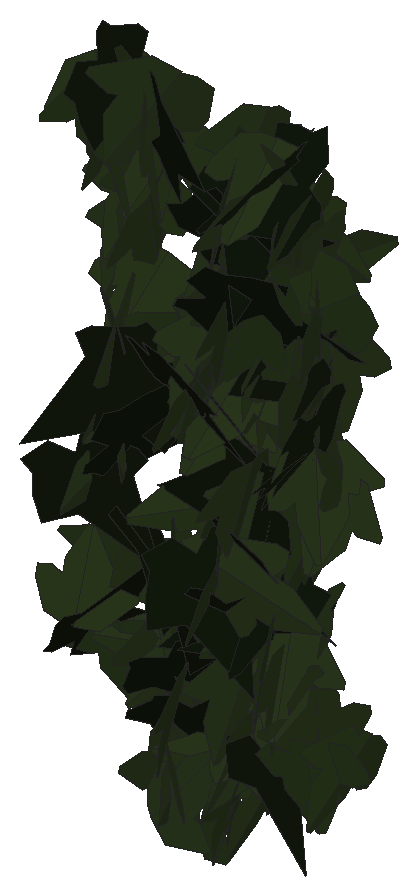
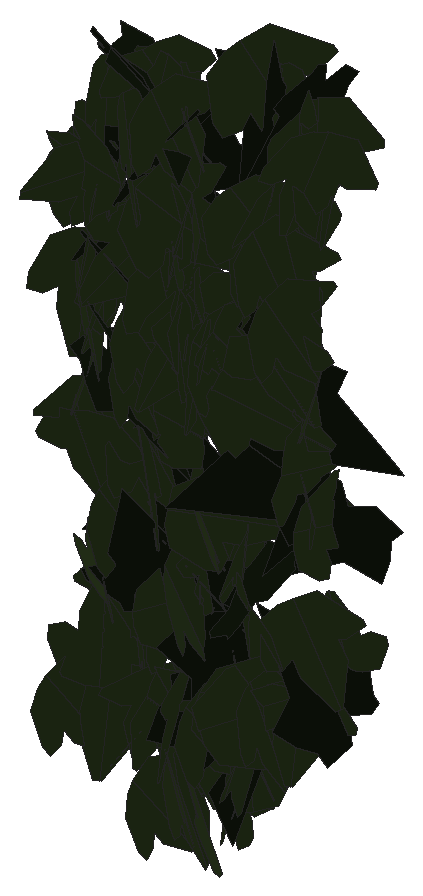
# SketchUp Ruby script. Lengths in inches.
U = 1.inch
M = Sketchup.active_model
def pt(a) = Geom::Point3d.new(a.map { |v| v * U })
def face(e, loops, mat)
  f = e.add_face(loops[0].map { |a| pt(a) })
  loops[1..].each { |l| e.add_face(l.map { |a| pt(a) }).erase! }
  f.material = f.back_material = mat if mat
  f
end
# faces: each face lists its corners as indices into pts; further lists are holes
def faces(e, pts, list, mat = nil) = list.each { |f| face(e, (f[0].is_a?(Array) ? f : [f]).map { |l| l.map { |i| pts[i] } }, mat) }
# xy, xz, yz: faces in a plane at the given z, y or x. An outline is a flat list of corners, or four numbers for a rectangle; further outlines are holes
def ring(l) = l.size == 4 ? [[l[0], l[1]], [l[2], l[1]], [l[2], l[3]], [l[0], l[3]]] : l.each_slice(2).to_a
def flat(e, list, mat, &to3) = list.each { |f| face(e, (f[0].is_a?(Array) ? f : [f]).map { |l| ring(l).map { |u, v| to3.(u, v) } }, mat) }
def xy(e, z, list, mat = nil) = flat(e, list, mat) { |x, y| [x, y, z] }
def xz(e, y, list, mat = nil) = flat(e, list, mat) { |x, z| [x, y, z] }
def yz(e, x, list, mat = nil) = flat(e, list, mat) { |y, z| [x, y, z] }
def lines(e, pts, list) = list.each { |a, b| e.add_line(pt(pts[a]), pt(pts[b])) }
# prism: a flat outline (further loops are holes) pulled along v
def prism(e, loops, v, mat = nil)
  f = face(e, loops, mat); d = Geom::Vector3d.new(v.map { |x| x * U })
  f.pushpull(f.normal.samedirection?(d) ? d.length : -d.length)
end
def box(e, o, s, mat = nil) = prism(e, [[o, [o[0] + s[0], o[1], o[2]], [o[0] + s[0], o[1] + s[1], o[2]], [o[0], o[1] + s[1], o[2]]]], [0, 0, s[2]], mat)
def at(x, y, z, deg = 0) = Geom::Transformation.translation(pt([x, y, z])) * Geom::Transformation.rotation(ORIGIN, Z_AXIS, deg.degrees)
def axes(o, x, y, z) = Geom::Transformation.new([*x, 0, *y, 0, *z, 0, *pt(o).to_a, 1])
def part(name) = M.definitions.add(name)
# library, detail: a bought-in or finely detailed component or shape, given as its bounding box
def library(name, o, s) = part(name).tap { |d| box(d.entities, o, s) }
def detail(e, o, s) = box(e.add_group.entities, o, s)
def put(e, d, t, mat = nil) = e.add_instance(d, t).tap { |i| i.material = mat if mat }
def group(e, t, mat = nil) = e.add_group.tap { |g| g.transformation = t; g.material = mat if mat }.entities
root = M.entities
M.materials.add("efeu1").color = [18, 25, 13]
M.materials.add("efeu2").color = [43, 57, 29]
c1 = part("ivyleaf_9")
p = [[1.54,2.16,1.25],[1.36,2.04,1.19],[-0.21,0.99,0.68],[-0.71,1.11,0.82],[-0.85,0.86,0.67],[-0.8,0.17,0.21],
  [-0.9,-0.01,0.1],[-0.67,-0.16,-0.02],[-0.08,-0.08,-0.05],[-0.03,-0.6,-0.4],[0.65,-0.88,-0.66],[0.83,-0.6,-0.49],
  [1.29,-0.42,-0.43],[1.8125,-0.07,-0.26],[1.21,0.44,0.15]]
faces(c1.entities,p,[[0,1,2,3,4,5,6,7,8,9,10,11,12,13,14]],"efeu1")
c2 = part("ivyleaf_10")
p = [[0,0.5,-0.03],[-0.0625,2.02,-0.43],[-0.19,2.01,-0.46],[-0.54,1.05,-0.29],[-0.52,0.625,-0.18],[-0.83,0.76,-0.28],
  [-1.16,0.64,-0.33],[-1.15,0.33,-0.24],[-0.77,-0.39,0.02],[-0.3,-0.51,0.16],[0.04,-0.48,0.23],[-0.02,2.01,-0.4375],
  [-0.06,2.01,-0.43],[0.04,-0.49,0.23],[0.67,-0.49,0.14],[1.38,0.36,-0.2],[1.375,0.51,-0.24],[0.81,0.65,-0.19],
  [0.62,0.59,-0.15],[0.6,1.09,-0.28],[0.5,1.23,-0.31]]
faces(c2.entities,p,[[0,1,2,3,4,5,6,7,8,9,10],[11,12,0,13,14,15,16,17,18,19,20]],"efeu2")
put(root,c1,axes([509.74,135.35,181.09],[0.74865,0.1371,0.35798],[0.34878,0.0823,-0.76093],[-0.15906,0.82575,0.0164]))
put(root,c2,axes([508.4,135.95,183.89],[-0.44907,-0.51344,0.43661],[-0.29886,-0.31855,-0.682],[0.6041,-0.53928,-0.01283]))
put(root,c2,axes([509.9375,135.84,177.97],[0.03708,-0.698,0.02112],[0.00383,-0.02095,-0.69898],[0.69831,0.03718,0.00271]))
put(root,c1,axes([509.16,135.75,176.39],[0.07993,-0.60102,-0.3989],[-0.03272,0.38262,-0.62961],[0.76932,0.07872,0.01466]))
put(root,c2,axes([509.58,136.01,182.89],[0.42901,-0.54847,0.24214],[0.15092,-0.18937,-0.69632],[0.58024,0.45477,0.00208]))
put(root,c1,axes([508.54,135.55,179.53],[0.80566,-0.10434,-0.13006],[-0.12795,0.02467,-0.81235],[0.10692,0.81571,0.00793]))
put(root,c2,axes([510.26,135.9375,175.45],[0.47005,-0.54569,0.14033],[0.14228,-0.06688,-0.72322],[0.59019,0.45073,0.06259]))
put(root,c1,axes([508.01,136.09,183.3],[0.34957,-0.1483,-0.68391],[0.69592,-0.00675,0.35718],[-0.07361,-0.76804,0.12891]))
put(root,c2,axes([510.26,135.95,183.33],[0.50117,0.37752,-0.27471],[-0.21702,-0.17155,-0.62212],[-0.4478,0.50565,-0.00596]))
put(root,c2,axes([509.875,135.82,176.33],[-0.25449,-0.01854,-0.67596],[0.66869,-0.11431,-0.24861],[-0.10057,-0.71317,0.05742]))
put(root,c2,axes([508.48,135.88,172.03],[0.5067,-0.23136,-0.42913],[0.39952,-0.15767,0.55673],[-0.27941,-0.64501,0.01783]))
put(root,c2,axes([509.73,136.06,174.59],[-0.1443,-0.64865,0.23347],[0.05381,-0.23727,-0.68215],[0.73935,-0.10933,0.09521]))
put(root,c2,axes([509.98,135.9,182.48],[-0.05674,-0.73413,-0.01355],[0.00167,0.01347,-0.73632],[0.73426,-0.05676,0.00063]))
put(root,c2,axes([508.56,136,173.99],[0.35158,-0.6314,0.07032],[0.05777,-0.04845,-0.73833],[0.68337,0.32893,0.02623]))
put(root,c2,axes([510,135.81,180.66],[-0.6448,0.01365,0.32318],[-0.3359,-0.03571,-0.61982],[0.00475,-0.67212,0.0395]))
put(root,c2,axes([509.08,136.29,179.8],[-0.20617,-0.56097,0.45342],[0.08723,-0.4875,-0.56348],[0.716,-0.10214,0.19921]))
put(root,c2,axes([509.51,135.63,176.35],[0.14705,-0.55935,-0.47093],[-0.10075,0.44324,-0.5986],[0.77068,0.16467,0.01161]))
put(root,c2,axes([509,135.76,179.13],[0.05501,-0.63551,-0.29193],[-0.01329,0.29183,-0.63779],[0.69923,0.05555,0.01084]))
put(root,c2,axes([509.64,135.97,180.82],[0.24546,-0.75777,-0.06924],[-0.0212,0.06591,-0.79653],[0.76063,0.24637,0.00014]))
put(root,c1,axes([509.63,135.77,175.78],[0.24193,0.5235,-0.42166],[-0.30427,-0.31199,-0.58083],[-0.64716,0.34239,0.11545]))
put(root,c1,axes([510.98,135.93,183.13],[-0.66132,0.32407,0.19389],[-0.17433,0.09353,-0.72048],[-0.3642,-0.63321,-0.00719]))
put(root,c2,axes([506.82,135.87,174.78],[0.53421,0.26987,-0.11623],[0.10494,0.05524,0.586],[0.29749,-0.50409,0.002]))
put(root,c2,axes([507.42,135.78,179.03],[0.28563,-0.46576,0.37687],[-0.19363,0.31491,0.55704],[-0.60721,-0.31952,-0.00036]))
put(root,c2,axes([507.21,135.99,183.4],[-0.39044,-0.55826,-0.05854],[0.04323,0.04114,-0.6916],[0.60443,-0.36356,0.01164]))
put(root,c1,axes([510.3125,135.54,182.98],[-0.01831,0.66027,0.3417],[-0.21376,0.31251,-0.66378],[-0.76728,-0.10282,0.17677]))
put(root,c2,axes([506.9375,136.49,177.05],[-0.00088,-0.1457,0.64268],[0.18114,-0.59606,-0.14593],[0.66134,0.16307,0.04083]))
put(root,c1,axes([506.8,135.9,177.2],[-0.16978,-0.17451,-0.6443],[0.4202,0.48225,-0.24395],[0.55373,-0.41946,-0.01243]))
put(root,c1,axes([507.75,136.4,178.85],[0.00594,0.02878,-0.77488],[-0.23754,-0.73758,-0.02921],[-0.73813,0.2376,0.00317]))
put(root,c1,axes([509.22,135.97,181.65],[0.25858,-0.12318,0.63865],[0.65506,-0.11834,-0.27062],[0.16868,0.6484,0.07194]))
put(root,c2,axes([508.18,136.5,172.11],[-0.09627,0.01251,0.69865],[0.44697,-0.53283,0.06743],[0.57165,0.41872,0.06493]))
put(root,c2,axes([507.8125,135.91,183.71],[0.52846,-0.33956,-0.35804],[-0.16665,0.37098,-0.5978],[0.46446,0.51946,0.19289]))
put(root,c1,axes([509.54,136.08,176.64],[0.63285,-0.2784,0.18541],[0.17991,-0.06473,-0.67457],[0.3084,0.60906,0.01305]))
put(root,c2,axes([508.4,136.23,176.26],[-0.15131,0.4737,-0.27839],[0.06779,-0.2605,-0.51359],[-0.58371,-0.15305,0.01252]))
put(root,c1,axes([509.62,136.6,182.33],[-0.03617,-0.73349,0.24261],[-0.01634,-0.2421,-0.73436],[0.77239,-0.03947,-0.00417]))
put(root,c2,axes([511,135.99,182.76],[0.04486,-0.66745,-0.25816],[0.03303,0.2501,-0.69404],[0.76837,0.02822,0.0449]))
put(root,c2,axes([507.03,136.47,177.33],[0.02375,-0.04227,-0.61922],[0.32303,-0.51483,0.0495],[-0.55788,-0.2999,0.0023]))
put(root,c2,axes([506.87,136.47,182.21],[0.0124,-0.4178,-0.42236],[0.00272,-0.40616,0.43463],[-0.62926,-0.00999,-0.00644]))
put(root,c1,axes([507.8,136.68,175.73],[-0.00325,-0.57717,0.50536],[0.21232,-0.48631,-0.55404],[0.73719,0.13752,0.1618]))
put(root,c2,axes([507.02,136.22,182.51],[-0.41747,0.30635,-0.30245],[0.2187,-0.21156,-0.51169],[-0.40036,-0.43501,0.03586]))
put(root,c1,axes([508.85,136.08,179.125],[0.66358,-0.25418,-0.01703],[-0.01545,0.00825,-0.69152],[0.27465,0.61459,0.00224]))
put(root,c2,axes([510.78,135.67,181.9],[-0.22226,0.28018,0.66253],[-0.3777,0.53271,-0.36115],[-0.64982,-0.40546,-0.01669]))
put(root,c1,axes([510,136.13,175.69],[-0.62619,0.34671,0.17629],[-0.1731,0.06196,-0.70197],[-0.37916,-0.60089,0.02933]))
put(root,c1,axes([507.27,135.85,183.93],[0.27219,-0.26955,-0.58781],[-0.25811,0.52174,-0.36961],[0.62509,0.33281,0.10334]))
put(root,c1,axes([510.02,136.17,177.49],[-0.21624,0.01699,-0.65577],[-0.60723,-0.30468,0.17714],[-0.3088,0.58724,0.11088]))
put(root,c2,axes([510.03,136.4,177.44],[-0.37029,-0.49175,0.32008],[-0.12959,-0.3006,-0.61174],[0.57226,-0.38627,0.06858]))
put(root,c2,axes([511.5,136.23,181.34],[-0.39534,-0.02108,0.59441],[-0.57469,-0.1704,-0.38827],[0.15328,-0.69324,0.07736]))
put(root,c2,axes([510.05,136.1,183.23],[-0.66301,0.21306,0.02845],[-0.02852,0.00734,-0.67581],[-0.23023,-0.61447,0.00179]))
put(root,c2,axes([508.52,136.04,172.71],[-0.35556,0.64282,0.07293],[-0.03912,0.0617,-0.73459],[-0.64576,-0.35768,0.00434]))
put(root,c2,axes([508.73,136.08,176.01],[0.1529,0.65572,0.10416],[0.02314,0.09784,-0.69766],[-0.71602,0.14318,-0.00031]))
put(root,c2,axes([508.19,136.37,172.41],[-0.27692,-0.6328,-0.06248],[-0.02477,-0.05553,0.71009],[-0.68605,0.25743,-0.00042]))
put(root,c2,axes([509.3,136.51,172.68],[0.08283,0.11746,0.59606],[-0.41295,-0.42744,0.14432],[0.47823,-0.38944,0.02138]))
put(root,c2,axes([509.38,136.44,179.29],[0.57693,0.31971,-0.32961],[-0.27891,-0.17649,-0.65937],[-0.36479,0.64058,-0.01716]))
put(root,c2,axes([510.1,136.39,174.68],[0.29758,-0.61754,0.07313],[0.15086,-0.01343,-0.69184],[0.65408,0.28405,0.12629]))
put(root,c2,axes([508.82,136.59,179.98],[0.4439,-0.40526,0.40246],[0.30385,-0.26403,-0.60102],[0.48361,0.53788,0.00821]))
put(root,c1,axes([506.64,136.13,174.06],[0.29306,0.60024,0.04948],[-0.04371,-0.03388,0.68466],[0.64882,-0.2734,0.02378]))
put(root,c2,axes([510.8,135.97,179.89],[0.10807,-0.46714,-0.52578],[0.0768,0.53661,-0.46098],[0.69912,0.01326,0.13191]))
put(root,c2,axes([510.26,136.38,175.06],[0.72295,0.16314,-0.00192],[-0.00094,-0.00425,-0.71654],[-0.1762,0.66938,-0.00408]))
put(root,c2,axes([508.83,136.61,176.87],[0.40752,-0.56305,0.27012],[0.13545,-0.23517,-0.69456],[0.60963,0.42864,-0.02624]))
put(root,c2,axes([509.65,136.62,173.34],[0.02303,0.47023,-0.48376],[-0.24457,-0.43208,-0.46506],[-0.67116,0.17359,0.15287]))
put(root,c2,axes([509.52,136.18,181.22],[-0.39493,0.49397,0.10178],[-0.0765,0.06929,-0.63898],[-0.53845,-0.37215,0.01613]))
put(root,c2,axes([509.48,136.51,181.22],[-0.09068,0.0637,-0.75894],[0.67885,-0.33974,-0.10962],[-0.34528,-0.68468,-0.01622]))
put(root,c2,axes([509.16,136.49,178.74],[0.5641,0.24317,-0.28606],[-0.26673,-0.1212,-0.59917],[-0.29339,0.57774,-0.00529]))
put(root,c2,axes([509.53,136.77,181.58],[-0.23767,-0.45278,0.56381],[-0.23283,-0.51396,-0.51089],[0.68461,-0.33198,0.02198]))
put(root,c1,axes([509.67,136.57,173.22],[0.28915,-0.62711,-0.01274],[0.00175,0.01401,-0.70911],[0.67741,0.26765,0.00727]))
put(root,c1,axes([510.88,136.56,179.44],[-0.62971,0.18788,-0.31806],[0.30825,-0.11107,-0.63687],[-0.23506,-0.64897,0.01692]))
put(root,c2,axes([509.5625,136.82,175],[-0.02297,-0.01876,0.60371],[-0.01107,-0.58078,-0.01991],[0.62716,-0.01094,0.02176]))
put(root,c2,axes([507.07,136.8125,178.15],[0.02837,0.21965,-0.61322],[-0.10492,-0.58166,-0.22985],[-0.67141,0.10018,0.01]))
put(root,c1,axes([508.7,136.18,173.55],[0.35472,0.51239,-0.32297],[-0.27921,-0.19828,-0.62461],[-0.58375,0.4062,0.1025]))
put(root,c2,axes([507.14,136.48,175.49],[-0.53092,-0.2481,0.33126],[-0.30883,-0.14034,-0.57267],[0.30782,-0.5687,-0.00319]))
put(root,c1,axes([510.68,136.39,178.57],[-0.43883,0.54711,-0.12384],[-0.0219,-0.1614,-0.69931],[-0.60431,-0.39144,0.11527]))
put(root,c2,axes([509.08,136.17,179.42],[0.06248,-0.58588,-0.42335],[0.00869,0.4255,-0.58759],[0.72278,0.04553,0.04366]))
put(root,c1,axes([508.44,136.03,174.39],[0.4233,0.5782,0.03835],[0.02564,0.02846,-0.72646],[-0.6252,0.39265,-0.00382]))
put(root,c1,axes([510.82,136.4,180.11],[-0.62436,0.31764,0.17042],[-0.14766,0.09138,-0.68587],[-0.35666,-0.5939,-0.01438]))
put(root,c2,axes([508.83,136.8125,176.77],[-0.12314,0.00717,0.69853],[-0.4244,-0.56416,-0.06903],[0.55487,-0.42991,0.10223]))
put(root,c2,axes([509.36,136.08,180.96],[0.09573,-0.0958,0.66685],[-0.51413,0.42972,0.13521],[-0.47533,-0.48409,-0.01195]))
put(root,c1,axes([507.53,135.84,177.72],[0.38353,0.33289,0.62618],[0.4278,0.45917,-0.50613],[-0.5656,0.57303,0.04179]))
put(root,c2,axes([511.01,136.16,180.92],[0.18054,-0.4942,-0.48629],[-0.00259,0.50203,-0.51115],[0.69333,0.13056,0.12472]))
put(root,c2,axes([510.69,136.64,173.67],[-0.44884,-0.46365,-0.10936],[-0.06153,-0.09009,0.6473],[-0.50976,0.41912,0.01816]))
put(root,c2,axes([507.84,136.69,175.46],[0.55016,-0.26282,0.35768],[0.32413,-0.15127,-0.6097],[0.30323,0.63853,0.00278]))
put(root,c2,axes([507.18,136.46,174.15],[-0.53897,-0.29968,-0.02889],[0.02564,0.01443,-0.6054],[0.32403,-0.49961,-0.00016]))
put(root,c2,axes([509.64,136.34,173.49],[0.35356,0.54241,0.22348],[0.12173,0.18741,-0.64746],[-0.57387,0.37393,0.00034]))
put(root,c2,axes([511.02,136.47,180.14],[-0.54851,-0.48159,-0.06748],[0.05353,0.04131,-0.72992],[0.48334,-0.5511,0.00426]))
put(root,c2,axes([510.87,136.8,178.1],[-0.31661,0.40704,0.46053],[0.28471,-0.35583,0.52167],[0.58388,0.39423,-0.00465]))
put(root,c2,axes([509.17,136.69,172.28],[0.16262,-0.64125,0.08728],[-0.00503,-0.08724,-0.68458],[0.69844,0.14868,-0.02525]))
put(root,c2,axes([510.2,136.9,176.47],[-0.01037,-0.6171,0.38591],[0.02914,-0.38599,-0.61645],[0.72725,0.00667,0.0302]))
put(root,c2,axes([509.39,136.83,183.1875],[-0.14289,-0.64037,0.27812],[0.03301,-0.28977,-0.65022],[0.69738,-0.11749,0.08776]))
put(root,c2,axes([506.91,136.53,179.42],[-0.37966,0.48175,-0.0988],[0.06135,-0.07616,-0.62023],[-0.52675,-0.3561,-0.00102]))
put(root,c2,axes([506.71,136.58,183.32],[-0.41406,-0.52131,-0.19237],[0.32099,-0.00433,-0.62798],[0.50384,-0.42566,0.24199]))
put(root,c2,axes([510.7,136.5625,178.11],[0.39491,0.5739,-0.00897],[0.00188,-0.01133,-0.70767],[-0.61988,0.36559,-0.00786]))
put(root,c2,axes([508.14,137.03,174.09],[-0.17752,-0.27541,0.58765],[-0.09901,-0.59062,-0.30671],[0.64139,-0.16739,0.1153]))
put(root,c2,axes([510.6,136.54,173.27],[-0.65332,-0.28186,-0.01273],[0.01368,0.00179,-0.69405],[0.30439,-0.60505,0.00387]))
put(root,c2,axes([508.4,137.04,179.72],[0.02504,-0.46652,0.54693],[0.25308,-0.50651,-0.44363],[0.67285,0.20787,0.14651]))
put(root,c2,axes([509.45,136.72,180.37],[-0.26004,-0.62676,0.10728],[-0.0288,-0.10417,-0.67843],[0.63522,-0.2613,0.01316]))
put(root,c2,axes([507.62,136.47,181.38],[0.01756,-0.64293,-0.28401],[0.01047,0.28431,-0.64295],[0.70279,0.01183,0.01668]))
put(root,c2,axes([507.42,136.8,181.51],[-0.54396,-0.26663,0.33121],[-0.217,-0.28168,-0.57574],[0.39259,-0.52512,0.14067]))
put(root,c2,axes([510.5,136.83,181.8],[-0.05423,0.0142,-0.67711],[0.58636,-0.35968,-0.0517],[-0.38838,-0.54501,0.01648]))
put(root,c2,axes([509.26,136.35,179.59],[-0.23114,-0.49201,-0.45452],[0.21124,0.40274,-0.54339],[0.63565,-0.31276,0.01531]))
put(root,c2,axes([508.34,136.89,179.91],[0.04851,0.41156,-0.39426],[-0.08531,-0.37185,-0.42957],[-0.59826,0.0864,0.02929]))
put(root,c2,axes([509.19,136.8,172.59],[0.36803,-0.54912,0.08981],[0.06082,-0.06667,-0.67198],[0.59725,0.34516,0.01308]))
put(root,c2,axes([508.54,136.8125,171.41],[0.42056,-0.45932,-0.32451],[0.23646,-0.22324,0.62242],[-0.51026,-0.48202,0.02097]))
put(root,c2,axes([509.92,136.43,180.83],[-0.4341,-0.28898,-0.47445],[0.38734,0.27417,-0.52139],[0.39821,-0.5817,-0.01005]))
put(root,c2,axes([508.01,136.84,179.01],[0.30173,0.17419,-0.66056],[-0.65139,-0.14423,-0.33557],[-0.20584,0.71174,0.09366]))
put(root,c2,axes([509.06,136.68,178.11],[-0.06814,-0.01687,0.7537],[0.74614,0.10671,0.06984],[-0.1078,0.74921,0.00703]))
put(root,c2,axes([509.71,136.99,179.64],[-0.0461,-0.61074,0.33039],[0.04486,-0.33304,-0.60939],[0.69293,-0.01907,0.06144]))
put(root,c2,axes([510.34,137.05,175.1875],[-0.04154,-0.25217,-0.57568],[0.30953,-0.49673,0.21463],[-0.57944,-0.24727,0.15592]))
put(root,c2,axes([508.12,136.72,173.1],[-0.4255,0.28219,-0.33037],[0.28792,-0.17316,-0.50384],[-0.35733,-0.47555,-0.01258]))
put(root,c2,axes([507.55,136.875,174.17],[0.0488,-0.67709,0.14502],[0.02266,-0.14374,-0.67874],[0.69207,0.05245,0.01199]))
put(root,c2,axes([507.52,136.76,182.4375],[-0.10181,0.58208,-0.13416],[0.02407,-0.12708,-0.61325],[-0.64345,-0.09685,-0.00171]))
put(root,c2,axes([507.72,137.0625,182.3125],[-0.44354,-0.37253,0.40167],[-0.13872,-0.42359,-0.54605],[0.52997,-0.42265,0.19322]))
put(root,c2,axes([510.83,136.77,179.86],[0.2659,-0.62103,-0.12277],[-0.04086,0.11604,-0.67551],[0.63173,0.2689,0.00798]))
put(root,c2,axes([511.01,137.1,173.26],[-0.09418,-0.53573,0.39099],[-0.03012,-0.39105,-0.54307],[0.66255,-0.09393,0.03089]))
put(root,c2,axes([510.92,136.23,181.57],[0.08374,-0.06374,0.73173],[0.01508,0.73646,0.06242],[-0.73434,0.00786,0.08472]))
put(root,c2,axes([508.91,137.08,175.75],[0.293,-0.62395,0.29477],[0.14627,-0.25681,-0.68899],[0.6744,0.32679,0.02137]))
put(root,c2,axes([508.4,137.17,173.71],[-0.03012,-0.53512,0.43757],[0.06973,-0.4381,-0.53098],[0.68772,0.02098,0.073]))
put(root,c2,axes([507.93,137.18,173.83],[0.09678,0.21341,0.70114],[-0.34188,-0.61242,0.23359],[0.64827,-0.35483,0.01852]))
put(root,c2,axes([507.39,136.9,180.04],[0.63235,0.14456,-0.26709],[-0.25719,-0.07321,-0.64853],[-0.16151,0.68252,-0.01299]))
put(root,c2,axes([510.04,136.75,182.81],[0.22164,-0.67623,-0.20192],[-0.04642,0.19722,-0.71143],[0.7042,0.22583,0.01665]))
put(root,c2,axes([509.34,136.52,173.54],[-0.25035,0.43182,0.34895],[-0.20994,0.27556,-0.5085],[-0.55203,-0.30063,0.03513]))
put(root,c1,axes([509.6,136.63,175.18],[-0.60138,-0.06605,0.45913],[0.46108,-0.00307,0.6035],[-0.05063,0.7566,0.04253]))
put(root,c2,axes([508.75,137.05,179.29],[-0.42493,0.20041,0.53617],[0.48869,-0.22066,0.46978],[0.29802,0.64757,-0.00585]))
put(root,c2,axes([509.35,137.2,172.2],[0.05088,-0.53477,0.39576],[0.04574,-0.39317,-0.53715],[0.66372,0.06809,0.00668]))
put(root,c2,axes([510.75,136.9,177.58],[0.70377,0.03778,-0.10763],[-0.1127,0.01258,-0.67857],[-0.03816,0.65968,0.0191]))
put(root,c2,axes([509.73,137.125,179.1],[0.0636,-0.62394,0.279],[0.10415,-0.26808,-0.62327],[0.67549,0.10008,0.06983]))
put(root,c2,axes([509.69,136.8,177.55],[0.42977,-0.51418,-0.19524],[-0.06182,0.20104,-0.66556],[0.54652,0.42708,0.07824]))
put(root,c2,axes([507.3,137.11,181.73],[-0.07527,-0.65296,0.24858],[0.00922,-0.25092,-0.65633],[0.69861,-0.06704,0.03544]))
put(root,c2,axes([506.98,137.2,180.84],[-0.1097,-0.58123,0.36956],[0.0552,-0.38043,-0.58195],[0.68655,-0.06229,0.10584]))
